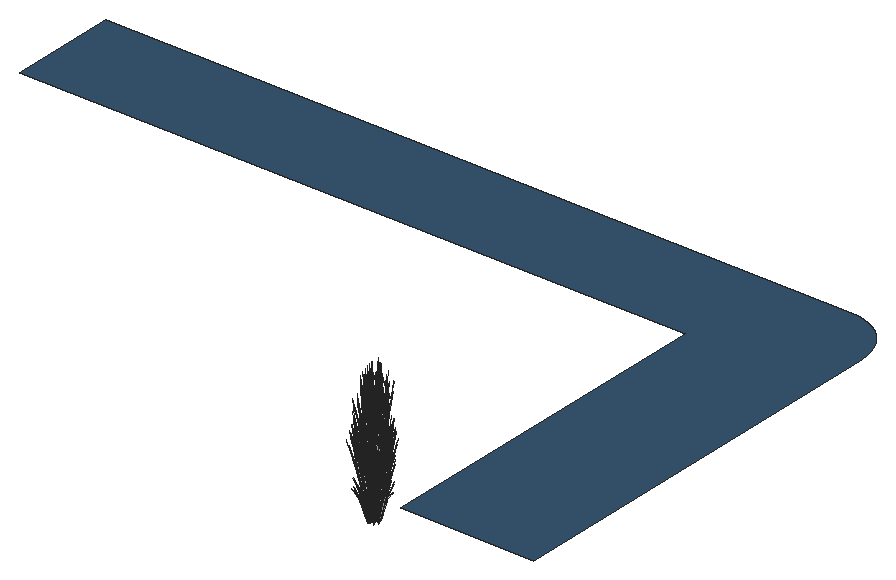
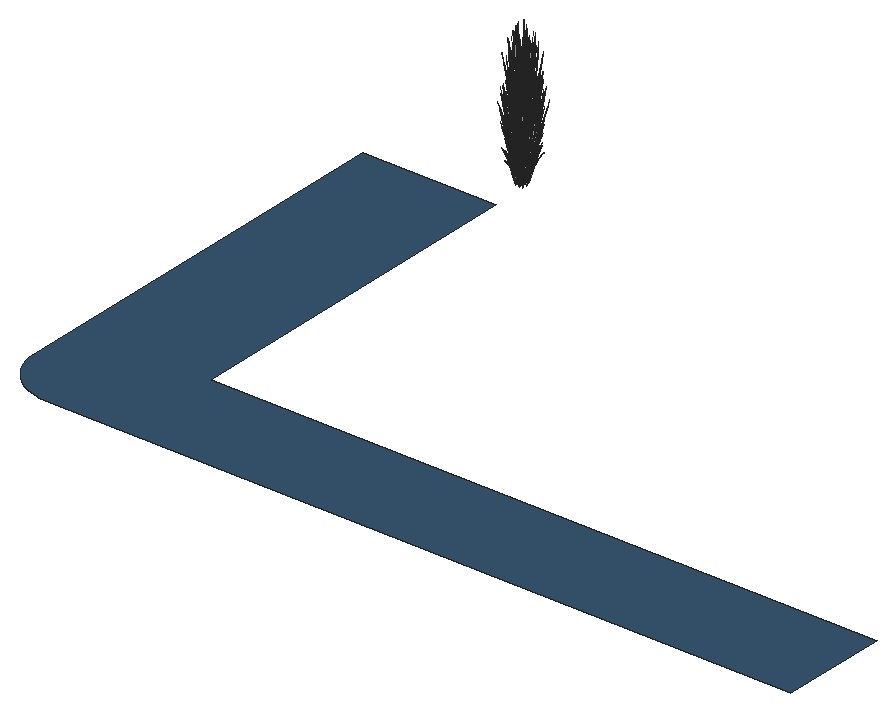
# SketchUp Ruby script. Lengths in inches.
U = 1.inch
M = Sketchup.active_model
def pt(a) = Geom::Point3d.new(a.map { |v| v * U })
def face(e, loops, mat)
  f = e.add_face(loops[0].map { |a| pt(a) })
  loops[1..].each { |l| e.add_face(l.map { |a| pt(a) }).erase! }
  f.material = f.back_material = mat if mat
  f
end
# faces: each face lists its corners as indices into pts; further lists are holes
def faces(e, pts, list, mat = nil) = list.each { |f| face(e, (f[0].is_a?(Array) ? f : [f]).map { |l| l.map { |i| pts[i] } }, mat) }
# xy, xz, yz: faces in a plane at the given z, y or x. An outline is a flat list of corners, or four numbers for a rectangle; further outlines are holes
def ring(l) = l.size == 4 ? [[l[0], l[1]], [l[2], l[1]], [l[2], l[3]], [l[0], l[3]]] : l.each_slice(2).to_a
def flat(e, list, mat, &to3) = list.each { |f| face(e, (f[0].is_a?(Array) ? f : [f]).map { |l| ring(l).map { |u, v| to3.(u, v) } }, mat) }
def xy(e, z, list, mat = nil) = flat(e, list, mat) { |x, y| [x, y, z] }
def xz(e, y, list, mat = nil) = flat(e, list, mat) { |x, z| [x, y, z] }
def yz(e, x, list, mat = nil) = flat(e, list, mat) { |y, z| [x, y, z] }
def lines(e, pts, list) = list.each { |a, b| e.add_line(pt(pts[a]), pt(pts[b])) }
# prism: a flat outline (further loops are holes) pulled along v
def prism(e, loops, v, mat = nil)
  f = face(e, loops, mat); d = Geom::Vector3d.new(v.map { |x| x * U })
  f.pushpull(f.normal.samedirection?(d) ? d.length : -d.length)
end
def box(e, o, s, mat = nil) = prism(e, [[o, [o[0] + s[0], o[1], o[2]], [o[0] + s[0], o[1] + s[1], o[2]], [o[0], o[1] + s[1], o[2]]]], [0, 0, s[2]], mat)
def at(x, y, z, deg = 0) = Geom::Transformation.translation(pt([x, y, z])) * Geom::Transformation.rotation(ORIGIN, Z_AXIS, deg.degrees)
def axes(o, x, y, z) = Geom::Transformation.new([*x, 0, *y, 0, *z, 0, *pt(o).to_a, 1])
def part(name) = M.definitions.add(name)
# library, detail: a bought-in or finely detailed component or shape, given as its bounding box
def library(name, o, s) = part(name).tap { |d| box(d.entities, o, s) }
def detail(e, o, s) = box(e.add_group.entities, o, s)
def put(e, d, t, mat = nil) = e.add_instance(d, t).tap { |i| i.material = mat if mat }
def group(e, t, mat = nil) = e.add_group.tap { |g| g.transformation = t; g.material = mat if mat }.entities
root = M.entities
M.materials.add("Carpet_04_1K").color = [56, 85, 112]
M.materials.add("LightPink_Translucent").color = [144, 107, 117]
M.materials["LightPink_Translucent"].alpha = 0.75
c1 = part("blade")
p = [[2.15,0.21,22],[0,0.17,0],[0.09,0.45,0],[2.18,0.31,22],[2.29,0.31,22],[0.38,0.45,0],
  [2.48,0.24,33],[2.49,0.24,33],[2.48,0.22,33]]
faces(c1.entities,p,[[0,1,2,3],[4,5,2,3],[6,3,4,7],[8,0,3,6]])
c2 = part("seeds")
p = [[0.3,-0.1,1.38],[-0.01,-0.03,1.59],[-0.01,-0.03,0.03],[0.14,-0.07,-0.07],[0.29,-0.03,3],[0.15,0.01,3.11]]
faces(c2.entities,p,[[0,1,2,3],[1,0,4,5]],"LightPink_Translucent")
c3 = part("blade with seeds")
put(c3.entities,c1,at(0,0,0))
put(c3.entities,c2,axes([2.4,0.25,30.99],[1.5799,-0.05474,1.17369],[-0.12525,1.92788,0.29478],[-0.07173,-0.02425,1.56792]))
xy(root,1398,[[330.57,637.9,390.57,637.9,390.57,822.7,390.37,825.83,389.76,828.91,388.75,831.89,387.36,834.7,385.62,837.3125,383.55,839.67,381.19,841.74,378.57,843.49,375.76,844.875,372.79,845.88,369.71,846.5,366.57,846.7,30.57,846.7,30.57,798.7,330.57,798.7]],"Carpet_04_1K")
put(root,c3,axes([332.43,620.08,1402.71],[-0.03584,0.03562,1.77383],[-0.35118,-0.12018,-0.16761],[-0.01271,-0.15545,0.31391]))
put(root,c3,axes([331.14,620.64,1402.68],[-0.34695,-0.11691,-0.51099],[0.11892,-0.40083,-0.3958],[-0.03181,-0.16138,0.97773]))
put(root,c3,axes([331.35,619.64,1400.77],[0.04528,0.27194,1.1486],[-0.25117,-0.15062,0.84392],[0.02703,-0.13924,0.25299]))
put(root,c3,axes([331.89,620.94,1402.68],[-0.25266,-0.31335,-0.51099],[0.2669,-0.27442,-0.3958],[0.03844,-0.15921,0.97773]))
put(root,c3,axes([330.52,619.4,1402.71],[-0.00658,0.0559,1.77383],[-0.32474,0.20287,-0.16761],[-0.09556,-0.1037,0.31391]))
put(root,c3,axes([330.45,620.39,1403.09],[0.39316,-0.11987,0.53763],[0.06823,0.47021,0.4433],[-0.09247,-0.13858,1.11249]))
put(root,c3,axes([331.34,620.48,1402.73],[0.34777,0.12192,0.48003],[-0.11892,0.40083,0.3958],[-0.0209,-0.15763,0.9933]))
put(root,c3,axes([331.4375,620.62,1403.03],[-0.34538,0.21713,-0.1216],[-0.16972,-0.38536,-0.67495],[-0.04557,-0.16239,1.02557]))
put(root,c3,axes([332.15,621.11,1403.03],[-0.3879,-0.02311,-0.1216],[0.0106,-0.43749,-0.67495],[0.02694,-0.1685,1.02557]))
put(root,c3,axes([332.13,620.83,1402.53],[0.23881,-0.24554,-0.35414],[0.22606,0.28036,0.4572],[0.0344,-0.14245,0.87481]))
put(root,c3,axes([330.0625,619.96,1400.77],[0.18411,0.16231,1.1486],[-0.26813,0.09757,0.84392],[-0.05737,-0.12474,0.25299]))
put(root,c3,axes([331.43,620.45,1402.73],[0.26007,-0.1585,0.0643],[0.12729,0.28902,0.50621],[-0.02512,-0.1274,0.77189]))
put(root,c3,axes([330.51,620.82,1402.98],[-0.30095,-0.22541,-0.71045],[0.21388,-0.395,0.08574],[-0.10904,-0.13459,1.00501]))
put(root,c3,axes([330.4,620.52,1402.53],[-0.05451,-0.37564,-0.35414],[0.31161,-0.09919,0.4572],[-0.0837,-0.10765,0.87481]))
put(root,c3,axes([330.54,620.49,1402.73],[0.16041,-0.29625,0.0643],[0.22843,0.17248,0.50621],[-0.07385,-0.09498,0.77189]))
put(root,c3,axes([329.92,620.45,1399.49],[-0.03419,0.06144,1.76342],[-0.3455,0.13246,-0.26939],[-0.08346,-0.12049,0.30037]))
put(root,c3,axes([330.49,622.14,1400.1],[-0.14494,-0.47823,-0.69835],[0.41752,-0.17223,-0.18329],[-0.01602,-0.16194,1.54149]))
put(root,c3,axes([329.73,621.07,1401.875],[0.1311,0.08035,1.71376],[-0.27131,0.33708,0.13857],[-0.16909,-0.15206,0.73262]))
put(root,c3,axes([332.43,620.68,1399.49],[-0.05283,-0.03674,1.76342],[-0.13569,-0.41045,-0.26939],[0.09154,-0.11138,0.30037]))
put(root,c3,axes([331.33,620.77,1403.05],[-0.1064,0.35863,0.35414],[-0.31043,-0.1046,-0.4572],[-0.02846,-0.14439,0.87481]))
put(root,c3,axes([330.37,620.83,1402.68],[-0.34827,0.11086,-0.51099],[-0.06092,-0.41983,-0.3958],[-0.09354,-0.12031,0.97773]))
put(root,c3,axes([332.125,620.92,1402.73],[0.25132,0.3182,0.48003],[-0.2669,0.27442,0.3958],[0.04636,-0.14929,0.9933]))
put(root,c3,axes([330.61,620.46,1403.43],[-0.23555,0.44708,-0.13619],[-0.34112,-0.25757,-0.75594],[-0.11858,-0.12631,1.14864]))
put(root,c3,axes([332.22,620.95,1402.73],[0.29004,0.02173,0.0643],[-0.00795,0.32812,0.50621],[0.03035,-0.12569,0.77189]))
put(root,c3,axes([332,621.17,1403.05],[-0.23881,0.24554,0.35414],[-0.22606,-0.28036,-0.4572],[0.0344,-0.14245,0.87481]))
put(root,c3,axes([332.42,621.84,1402.98],[0.18436,-0.36797,-0.71045],[0.32306,0.26151,0.08574],[0.11008,-0.13332,1.00501]))
put(root,c3,axes([330.43,620.76,1400.375],[-0.22066,-0.46731,0],[0.36918,-0.26061,-0.51607],[0.08408,-0.05936,1.63711]))
put(root,c3,axes([332.41,621.66,1402.68],[-0.09067,-0.42583,-0.51099],[0.34336,-0.07449,-0.3958],[0.0984,-0.11438,0.97773]))
put(root,c3,axes([330.92,620.2,1400.13],[-0.2439,0.26754,-0.03893],[-0.22348,-0.29302,-0.17649],[-0.01573,-0.08303,0.58215]))
put(root,c3,axes([329.71,620.33,1402.72],[-0.07594,-0.00329,1.74944],[-0.24177,0.32918,-0.27667],[-0.129,-0.06726,0.14031]))
put(root,c3,axes([332.58,621.97,1403.03],[-0.32648,-0.25715,-0.1216],[0.18809,-0.3724,-0.67495],[0.09224,-0.12945,1.02557]))
put(root,c3,axes([331.23,623.37,1401.33],[0.305,0.18805,1.51261],[-0.29879,0.40513,0.59816],[-0.13384,-0.24012,1.26806]))
put(root,c3,axes([330.59,620.83,1403.05],[0.05451,0.37564,0.35414],[-0.31161,0.09919,-0.4572],[-0.0837,-0.10765,0.87481]))
put(root,c3,axes([329.63,622.07,1400.02],[0,-0.46636,-0.49651],[0.39487,0,0],[0,-0.10622,1.57504]))
put(root,c3,axes([330.73,620.69,1400.02],[0.33032,-0.23318,-0.49651],[0.19744,0.41812,0],[0.07523,-0.05311,1.57504]))
put(root,c3,axes([332.69,621.5,1400.59],[-0.12609,-0.01381,1.43002],[-0.12917,-0.37055,-0.30754],[0.1549,-0.10482,0.61141]))
put(root,c3,axes([329.65,621.08,1403.09],[0.29147,-0.34417,0.53763],[0.25138,0.3655,0.4433],[-0.13675,-0.06349,1.11249]))
put(root,c3,axes([333.38,621.86,1402.71],[-0.0461,-0.00354,1.77383],[-0.19143,-0.37951,-0.16761],[0.07688,-0.12478,0.31391]))
put(root,c3,axes([331.12,621.65,1400.06],[0.23773,-0.35053,-0.62353],[0.29532,0.31785,-0.16365],[0.09526,-0.08744,1.37633]))
put(root,c3,axes([332.84,620.82,1400.77],[-0.11756,0.2374,1.1486],[-0.10105,-0.31895,0.84392],[0.09709,-0.07992,0.25299]))
put(root,c3,axes([332.67,621.71,1402.53],[0.30722,-0.06665,-0.35414],[0.08112,0.381,0.4572],[0.08804,-0.10234,0.87481]))
put(root,c3,axes([329.78,621.07,1402.73],[0.01777,-0.35463,0.0643],[0.26836,0.00972,0.50621],[-0.1028,-0.03711,0.77189]))
put(root,c3,axes([330.71,622.26,1400.21],[0.17124,-0.42022,-0.44739],[0.35581,0.20224,0.21531],[0,-0.09687,1.43643]))
put(root,c3,axes([329.68,621.19,1402.53],[-0.20082,-0.29199,-0.35414],[0.2293,-0.2764,0.4572],[-0.1165,-0.04206,0.87481]))
put(root,c3,axes([330.86,622.06,1400.67],[-0.04113,-0.53214,-0.29095],[0.42835,-0.03218,-0.50002],[0.07543,-0.07088,1.59708]))
put(root,c3,axes([329.8,622.08,1400.03],[0.24637,-0.29097,-0.30978],[0.24637,0.29097,0.30978],[0,-0.09372,1.38974]))
put(root,c3,axes([329.7,620.6875,1400.13],[-0.10181,0.3808,-0.03893],[-0.31336,-0.11714,-0.17649],[-0.04758,-0.06228,0.58215]))
put(root,c3,axes([332.42,621.93,1403.05],[-0.30722,0.06665,0.35414],[-0.08112,-0.381,-0.4572],[0.08804,-0.10234,0.87481]))
put(root,c3,axes([330.67,622.61,1400.67],[-0.39748,-0.22252,-0.29095],[0.19139,-0.46966,-0.50002],[-0.01249,-0.11531,1.59708]))
put(root,c3,axes([329.53,622.43,1400.375],[-0.44133,0,0],[0,-0.52122,-0.51607],[0,-0.11871,1.63711]))
put(root,c3,axes([329.61,621.5,1400.59],[0.06891,0.12984,1.43002],[-0.15879,0.35293,-0.30754],[-0.16304,-0.08436,0.61141]))
put(root,c3,axes([330.81,620.875,1400.03],[0.32928,0.11539,-0.30978],[-0.08291,0.40636,0.30978],[0.06638,-0.04686,1.38974]))
put(root,c3,axes([329.89,621.38,1402.98],[-0.35281,-0.01123,-0.71045],[0.0237,-0.47284,0.08574],[-0.14947,-0.0499,1.00501]))
put(root,c3,axes([332.7,621.875,1402.73],[0.2423,0.19613,0.0643],[-0.14107,0.2793,0.50621],[0.07768,-0.0903,0.77189]))
put(root,c3,axes([332.63,621.79,1402.73],[0.08753,0.42921,0.48003],[-0.34336,0.07449,0.3958],[0.1012,-0.10094,0.9933]))
put(root,c3,axes([333.55,622.3125,1402.72],[0.04898,-0.07104,1.74944],[-0.06269,-0.43574,-0.27667],[0.12289,-0.08262,0.14031]))
put(root,c3,axes([329.875,622.29,1400.33],[-0.32829,0.39208,0.30756],[-0.32849,-0.38796,-0.36492],[-0.01146,-0.11134,1.64885]))
put(root,c3,axes([329.42,620.61,1402.71],[0.02617,0.04654,1.77383],[-0.12614,0.41836,-0.16761],[-0.12775,0.00303,0.31391]))
put(root,c3,axes([330.92,622.47,1400.43],[0.39767,0.22603,0.24065],[-0.19139,0.46966,0.50002],[0,-0.10827,1.60543]))
put(root,c3,axes([330.77,623.11,1400.4375],[0.09355,-0.55261,-0.23429],[0.44354,0.09633,0.51271],[-0.0775,-0.07631,1.5644]))
put(root,c3,axes([329.78,621.48,1402.68],[-0.25628,0.30892,-0.51099],[-0.22444,-0.32634,-0.3958],[-0.13021,-0.047,0.97773]))
put(root,c3,axes([329.97,621.34,1403.05],[0.20082,0.29199,0.35414],[-0.2293,0.2764,-0.4572],[-0.1165,-0.04206,0.87481]))
put(root,c3,axes([329.2,621.89,1400.77],[0.22533,-0.03337,1.1486],[-0.14293,0.29403,0.84392],[-0.11135,-0.04411,0.25299]))
put(root,c3,axes([330.79,622.16,1400.72],[-0.38326,0.02879,0.44739],[-0.03466,-0.47788,-0.21531],[0.06861,-0.04843,1.43643]))
put(root,c3,axes([329.91,621.15,1403.03],[-0.0189,0.47427,-0.1216],[-0.35781,-0.01296,-0.67495],[-0.13781,-0.03295,1.02557]))
put(root,c3,axes([329.8,622.51,1400.48],[0,0.46636,0.49651],[-0.39487,0,0],[0,-0.10622,1.57504]))
put(root,c3,axes([332.59,622.97,1403.03],[-0.17758,-0.42229,-0.1216],[0.31518,-0.20752,-0.67495],[0.13282,-0.05572,1.02557]))
put(root,c3,axes([332.57,622.61,1402.68],[0.09562,-0.42421,-0.51099],[0.32782,0.1454,-0.3958],[0.13199,-0.0389,0.97773]))
put(root,c3,axes([332.06,620.88,1400.375],[0.22066,-0.46731,0],[0.36918,0.26061,-0.51607],[0.08408,0.05936,1.63711]))
put(root,c3,axes([329.46,621.81,1401.875],[0.14639,-0.01056,1.71376],[-0.09712,0.45778,0.13857],[-0.20862,-0.02831,0.73262]))
put(root,c3,axes([330.73,622.88,1400.21],[-0.21202,-0.39143,-0.44739],[0.32115,-0.27564,0.21531],[-0.06861,-0.04843,1.43643]))
put(root,c3,axes([330.78,622.33,1400.36],[0.15345,0.52148,0.45755],[-0.43845,0.18134,0.17955],[0.00536,-0.09582,1.58856]))
put(root,c3,axes([332.92,622.73,1399.98],[-0.22732,0.05597,1.41583],[-0.03618,-0.44548,0.08104],[0.15921,-0.06743,0.80566]))
put(root,c3,axes([333.34,622.33,1400.26],[-0.21881,-0.29821,-0.06488],[0.23965,-0.27324,-0.29416],[0.0679,-0.01924,0.97024]))
put(root,c3,axes([330.7,622.74,1400.72],[-0.17124,0.42022,0.44739],[-0.35581,-0.20224,-0.21531],[0,-0.09687,1.43643]))
put(root,c3,axes([331.33,622.375,1400.21],[0,-0.53961,0],[0.44133,0,0],[0,0,1.79456]))
put(root,c3,axes([331.87,621.125,1400.48],[-0.33032,-0.23318,0.49651],[0.19744,-0.41812,0],[0.07523,0.05311,1.57504]))
put(root,c3,axes([332.51,622.76,1402.98],[0.31014,-0.20596,-0.71045],[0.17284,0.42397,0.08574],[0.14985,-0.04816,1.00501]))
put(root,c3,axes([330.54,623.03,1400.06],[-0.36714,-0.07646,-0.62353],[0.07747,-0.47163,-0.16365],[-0.10956,-0.05715,1.37633]))
put(root,c3,axes([331.12,622.03,1400.36],[-0.29264,0.42323,0.45755],[-0.34767,-0.3736,0.17955],[0.07055,-0.04224,1.58856]))
put(root,c3,axes([331.44,622.79,1400.3],[-0.32829,-0.4014,-0.06131],[0.32849,-0.40164,0],[-0.01146,-0.01402,1.75571]))
put(root,c3,axes([330.61,621.34,1400.47],[-0.10196,0.46348,0.17642],[-0.3731,-0.13116,0.35086],[0.06445,-0.00226,1.60407]))
put(root,c3,axes([332.47,622.85,1403.05],[-0.29332,-0.1301,0.35414],[0.08555,-0.37955,-0.4572],[0.11809,-0.0348,0.87481]))
put(root,c3,axes([329.4,622.15,1402.73],[0.09971,-0.42522,0.48003],[0.32782,0.1454,0.3958],[-0.12892,0.02555,0.9933]))
put(root,c3,axes([330.46,621.71,1399.59],[-0.3474,0.18671,1.28929],[-0.11057,-0.53572,0.50096],[0.21332,0.00891,1.46642]))
put(root,c3,axes([331.39,621.85,1400.62],[0.06809,-0.4162,0.1448],[0.33266,0.07225,-0.41347],[0.06054,0.04274,1.26744]))
put(root,c3,axes([329.37,622.04,1402.73],[-0.12963,-0.31798,0.0643],[0.23638,-0.15564,0.50621],[-0.1042,0.03071,0.77189]))
put(root,c3,axes([330.82,622.84,1400.36],[0.44609,0.09826,0.45755],[-0.09078,0.55493,0.17955],[-0.06519,-0.05359,1.58856]))
put(root,c3,axes([333.17,622.4375,1399.49],[-0.01845,-0.0708,1.76342],[0.12793,-0.41416,-0.26939],[0.12905,-0.00596,0.30037]))
put(root,c3,axes([329.36,622.37,1399.49],[0.00895,0.0735,1.76342],[-0.18044,0.38382,-0.26939],[-0.12817,-0.01935,0.30037]))
put(root,c3,axes([331.25,621.96,1400.72],[-0.21202,-0.39143,0.44739],[0.32115,-0.27564,-0.21531],[0.06861,0.04843,1.43643]))
put(root,c3,axes([330.15,623.75,1400.03],[-0.08291,-0.40636,-0.30978],[0.32928,-0.11539,0.30978],[-0.06638,-0.04686,1.38974]))
put(root,c3,axes([330.58,623.73,1400.47],[0.37926,-0.12378,0.17642],[0.09365,0.46065,0.35086],[-0.03382,-0.06712,1.60407]))
put(root,c3,axes([331.36,621.99,1400.67],[0.35635,-0.30962,-0.29095],[0.23697,0.43749,-0.50002],[0.08792,0.04443,1.59708]))
put(root,c3,axes([332.78,622.8,1402.53],[0.29332,0.1301,-0.35414],[-0.08555,0.37955,0.4572],[0.11809,-0.0348,0.87481]))
put(root,c3,axes([330.0625,623.92,1400.02],[-0.33032,-0.23318,-0.49651],[0.19744,-0.41812,0],[-0.07523,-0.05311,1.57504]))
put(root,c3,axes([332.26,621.16,1400.02],[0.33032,0.23318,-0.49651],[-0.19744,0.41812,0],[0.07523,0.05311,1.57504]))
put(root,c3,axes([329.33,622.2,1402.53],[-0.29332,-0.1301,-0.35414],[0.08555,-0.37955,0.4572],[-0.11809,0.0348,0.87481]))
put(root,c3,axes([331.63,622.49,1400.21],[0.39487,0,0],[0,0.48281,0],[0,0,1.78407]))
put(root,c3,axes([330.96,623.1,1400.67],[-0.35635,0.30962,-0.29095],[-0.23697,-0.43749,-0.50002],[-0.08792,-0.04443,1.59708]))
put(root,c3,axes([331.74,621.36,1400.47],[-0.37926,0.12378,0.17642],[-0.09365,-0.46065,0.35086],[0.03382,0.06712,1.60407]))
put(root,c3,axes([331.98,622.33,1401.875],[-0.14639,0.01056,1.71376],[0.09712,-0.45778,0.13857],[0.20862,0.02831,0.73262]))
put(root,c3,axes([332.17,621.34,1400.03],[0.08291,0.40636,-0.30978],[-0.32928,0.11539,0.30978],[0.06638,0.04686,1.38974]))
put(root,c3,axes([332.73,622.96,1402.73],[0.12963,0.31798,0.0643],[-0.23638,0.15564,0.50621],[0.1042,-0.03071,0.77189]))
put(root,c3,axes([331.5,622.25,1400.38],[-0.44609,-0.09826,0.49198],[0.09078,-0.55493,0.19306],[0.06519,0.05359,1.70813]))
put(root,c3,axes([332.71,622.85,1402.73],[-0.09971,0.42522,0.48003],[-0.32782,-0.1454,0.3958],[0.12892,-0.02555,0.9933]))
put(root,c3,axes([331.15,623.62,1400.2],[-0.11516,-0.40207,0],[0.32884,-0.1408,0],[0,0,1.54371]))
put(root,c3,axes([330.93,623.24,1400.62],[-0.06809,0.4162,0.1448],[-0.33266,-0.07225,-0.41347],[-0.06054,-0.04274,1.26744]))
put(root,c3,axes([329.64,622.16,1403.05],[0.29332,0.1301,0.35414],[-0.08555,0.37955,-0.4572],[-0.11809,0.0348,0.87481]))
put(root,c3,axes([331.58,623.5625,1400.18],[0.37054,-0.15823,-0.19198],[0.1302,0.45581,0.00008],[0.0409,-0.01749,1.73897]))
put(root,c3,axes([331.71,623.75,1400.47],[0.10196,-0.46348,0.17642],[0.3731,0.13116,0.35086],[-0.06445,0.00226,1.60407]))
put(root,c3,axes([331.62,622.7,1400.21],[0.24637,0.30123,0],[-0.24637,0.30123,0],[0,0,1.69266]))
put(root,c3,axes([330.22,622.14,1401.34],[0.10032,-0.06746,1.77064],[0.0346,0.47103,0.13857],[-0.2173,0.0625,0.63284]))
put(root,c3,axes([332.29,622.57,1400.47],[-0.2773,-0.3397,0.17642],[0.27945,-0.32949,0.35086],[-0.03063,0.06937,1.60407]))
put(root,c3,axes([331.78,622.06,1400.06],[0.36714,0.07646,-0.62353],[-0.07747,0.47163,-0.16365],[0.10956,0.05715,1.37633]))
put(root,c3,axes([333.4,622.88,1400.77],[-0.21807,0.07699,1.1486],[0.10265,-0.31819,0.84392],[0.11568,0.02177,0.25299]))
put(root,c3,axes([331.07,623.8,1400.2],[-0.35581,-0.20937,0],[0.17124,-0.43505,0],[0,0,1.62707]))
put(root,c3,axes([331.36,623.24,1400.46],[-0.34464,-0.37536,-0.25192],[0.29,-0.42149,0.5513],[-0.0928,0.04391,1.68216]))
put(root,c3,axes([330.45,623.96,1400.48],[0.33032,0.23318,0.49651],[-0.19744,0.41812,0],[-0.07523,-0.05311,1.57504]))
put(root,c3,axes([331.62,622.35,1400.72],[0.17124,-0.42022,0.44739],[0.35581,0.20224,-0.21531],[0,0.09687,1.43643]))
put(root,c3,axes([333.3,624.23,1402.71],[-0.03191,-0.04083,1.77383],[0.06981,-0.43764,-0.16761],[0.12571,-0.02796,0.31391]))
put(root,c3,axes([329.14,622.45,1402.72],[-0.05763,0.06055,1.74944],[0.0049,0.44239,-0.27667],[-0.13211,0.05753,0.14031]))
put(root,c3,axes([331.55,622.59,1400.29],[0,0.53934,-0.05637],[-0.44133,0,0],[0,0.01695,1.79368]))
put(root,c3,axes([329.53,622.39,1402.68],[-0.09562,0.42421,-0.51099],[-0.32782,-0.1454,-0.3958],[-0.13199,0.0389,0.97773]))
put(root,c3,axes([329.51,622.03,1403.03],[0.17758,0.42229,-0.1216],[-0.31518,0.20752,-0.67495],[-0.13282,0.05572,1.02557]))
put(root,c3,axes([331.58,622.21,1400.21],[0.21202,0.39143,-0.44739],[-0.32115,0.27564,0.21531],[0.06861,0.04843,1.43643]))
put(root,c3,axes([333.02,623.86,1401.93],[-0.06755,-0.39203,-0.03492],[0.31928,-0.09013,-0.15832],[0.06667,0.02485,0.52218]))
put(root,c3,axes([330.26,624.21,1400.375],[-0.22066,0.46731,0],[-0.36918,-0.26061,-0.51607],[-0.08408,-0.05936,1.63711]))
put(root,c3,axes([332.19,623.85,1403.03],[0.0189,-0.47427,-0.1216],[0.35781,0.01296,-0.67495],[0.13781,0.03295,1.02557]))
put(root,c3,axes([332.52,622.58,1400.48],[0,-0.46636,0.49651],[0.39487,0,0],[0,0.10622,1.57504]))
put(root,c3,axes([331.53,622.93,1400.72],[0.38326,-0.02879,0.44739],[0.03466,0.47788,-0.21531],[-0.06861,0.04843,1.43643]))
put(root,c3,axes([331.77,622.44,1400.62],[0.32884,-0.136,0.1448],[0.11516,0.38837,-0.41347],[0,0.08547,1.26744]))
put(root,c3,axes([332.14,623.66,1403.05],[-0.20082,-0.29199,0.35414],[0.2293,-0.2764,-0.4572],[0.1165,0.04206,0.87481]))
put(root,c3,axes([331.1875,623.16,1400.21],[-0.38326,0.02879,-0.44739],[-0.03466,-0.47788,0.21531],[-0.06861,0.04843,1.43643]))
put(root,c3,axes([332.99,623.39,1400.59],[-0.085,-0.1147,1.43002],[0.1106,-0.37943,-0.30754],[0.17198,0.0514,0.61141]))
put(root,c3,axes([331.47,623.81,1400.2],[0.35581,0.20937,0],[-0.17124,0.43505,0],[0,0,1.74954]))
put(root,c3,axes([332.5,623.57,1402.72],[0.07571,-0.00789,1.74944],[0.20767,-0.36231,-0.27667],[0.13467,0.04783,0.14031]))
put(root,c3,axes([331.61,624.27,1400.19],[-0.21791,-0.46895,-0.05142],[0.36918,-0.26061,0.51607],[-0.09097,0.04465,1.6363]))
put(root,c3,axes([331.53,623.14,1400.62],[0.26075,0.2802,0.1448],[-0.2175,0.31612,-0.41347],[-0.06054,0.04274,1.26744]))
put(root,c3,axes([329.47,623.21,1402.73],[-0.08753,-0.42921,0.48003],[0.34336,-0.07449,0.3958],[-0.1012,0.10094,0.9933]))
put(root,c3,axes([329.41,623.13,1402.73],[-0.2423,-0.19613,0.0643],[0.14107,-0.2793,0.50621],[-0.07768,0.0903,0.77189]))
put(root,c3,axes([329.52,622.61,1401.875],[0.12246,-0.09864,1.71376],[0.1031,0.45582,0.13857],[-0.19225,0.10302,0.73262]))
put(root,c3,axes([332.21,623.62,1402.98],[0.35281,0.01123,-0.71045],[-0.0237,0.47284,0.08574],[0.14947,0.0499,1.00501]))
put(root,c3,axes([331.8125,624,1400.48],[0.33032,-0.23318,0.49651],[0.19744,0.41812,0],[-0.07523,0.05311,1.57504]))
put(root,c3,axes([331.34,623.63,1400.29],[0.15345,0.53576,-0.06012],[-0.43845,0.18773,0],[0.00536,0.01871,1.72173]))
put(root,c3,axes([331.51,624.21,1400.03],[-0.32928,-0.11539,-0.30978],[0.08291,-0.40636,0.30978],[-0.06638,0.04686,1.38974]))
put(root,c3,axes([329.14,623.39,1400.59],[0.12266,0.03828,1.43002],[0.07906,0.39104,-0.30754],[-0.16661,0.0732,0.61141]))
put(root,c3,axes([329.6875,623.07,1403.05],[0.30722,-0.06665,0.35414],[0.08112,0.381,-0.4572],[-0.08804,0.10234,0.87481]))
put(root,c3,axes([332.78,622.66,1400.375],[0.44133,0,0],[0,0.52122,-0.51607],[0,0.11871,1.63711]))
put(root,c3,axes([328.5,622.9,1402.71],[0.04504,0.01251,1.77383],[0.13934,0.41205,-0.16761],[-0.0922,0.10815,0.31391]))
put(root,c3,axes([332.61,622.93,1400.2],[-0.44111,-0.00373,-0.04976],[0,-0.52122,0.49943],[-0.01386,0.11865,1.58352]))
put(root,c3,axes([331.65,622.48,1400.67],[0.39748,0.22252,-0.29095],[-0.19139,0.46966,-0.50002],[0.01249,0.11531,1.59708]))
put(root,c3,axes([328.88,624.21,1400.77],[0.14709,-0.21136,1.1486],[0.05804,0.3346,0.84392],[-0.1063,0.05991,0.25299]))
put(root,c3,axes([332.42,623.82,1402.53],[0.20082,0.29199,-0.35414],[-0.2293,0.2764,0.4572],[0.1165,0.04206,0.87481]))
put(root,c3,axes([332.52,623.01,1400.03],[-0.24637,0.29097,-0.30978],[-0.24637,-0.29097,0.30978],[0,0.09372,1.38974]))
put(root,c3,axes([331.46,623.03,1400.67],[0.04113,0.53214,-0.29095],[-0.42835,0.03218,-0.50002],[-0.07543,0.07088,1.59708]))
put(root,c3,axes([332.32,623.93,1402.73],[-0.01777,0.35463,0.0643],[-0.26836,-0.00972,0.50621],[0.1028,0.03711,0.77189]))
put(root,c3,axes([331.61,622.83,1400.21],[-0.17124,0.42022,-0.44739],[-0.35581,-0.20224,0.21531],[0,0.09687,1.43643]))
put(root,c3,axes([329.43,623.29,1402.53],[-0.30722,0.06665,-0.35414],[-0.08112,-0.381,0.4572],[-0.08804,0.10234,0.87481]))
put(root,c3,axes([332.34,623.82,1402.73],[-0.26024,0.30729,0.48003],[-0.22444,-0.32634,0.3958],[0.1221,0.05668,0.9933]))
put(root,c3,axes([328.99,624.15,1403.65],[0.31145,0.12449,-0.06488],[-0.0958,0.38314,-0.29416],[-0.05094,0.05817,0.97024]))
put(root,c3,axes([331.2,623.44,1400.06],[-0.23773,0.35053,-0.62353],[-0.29532,-0.31785,-0.16365],[-0.09526,0.08744,1.37633]))
put(root,c3,axes([331.52,624.17,1403.05],[-0.05451,-0.37564,0.35414],[0.31161,-0.09919,-0.4572],[0.0837,0.10765,0.87481]))
put(root,c3,axes([331.62,624.03,1400.33],[0.44186,0.15158,0.30756],[-0.11054,0.54181,-0.36492],[-0.07313,0.06781,1.64885]))
put(root,c3,axes([331.59,624.4,1400.02],[-0.33032,0.23318,-0.49651],[-0.19744,-0.41812,0],[-0.07523,0.05311,1.57504]))
put(root,c3,axes([332.6875,623.02,1400.02],[0,0.46636,-0.49651],[-0.39487,0,0],[0,0.10622,1.57504]))
put(root,c3,axes([331.7,623.07,1401.875],[-0.1311,-0.08035,1.71376],[0.27131,-0.33708,0.13857],[0.16909,0.15206,0.73262]))
put(root,c3,axes([331.72,622.01,1402.47],[-0.30498,-0.24231,1.38283],[0.32203,-0.37727,0.59665],[0.0984,0.22736,1.33663]))
put(root,c3,axes([329.53,623.03,1403.03],[0.32648,0.25715,-0.1216],[-0.18809,0.3724,-0.67495],[-0.09224,0.12945,1.02557]))
put(root,c3,axes([332.18,623.98,1400.77],[-0.19872,-0.13409,1.1486],[0.2566,-0.13625,0.84392],[0.06921,0.11541,0.25299]))
put(root,c3,axes([331.49,624.37,1403.03],[0.21031,-0.39918,-0.1216],[0.30457,0.22997,-0.67495],[0.10587,0.11278,1.02557]))
put(root,c3,axes([329.97,622.92,1401.875],[0.08815,-0.14329,1.71376],[0.22258,0.38678,0.13857],[-0.15267,0.17614,0.73262]))
put(root,c3,axes([329.6875,623.34,1402.68],[0.09067,0.42583,-0.51099],[-0.34336,0.07449,-0.3958],[-0.0984,0.11438,0.97773]))
put(root,c3,axes([330.1,623.83,1403.05],[0.23881,-0.24554,0.35414],[0.22606,0.28036,-0.4572],[-0.0344,0.14245,0.87481]))
put(root,c3,axes([331.89,624.32,1400.375],[0.22066,0.46731,0],[-0.36918,0.26061,-0.51607],[-0.08408,0.05936,1.63711]))
put(root,c3,axes([331.21,624.7,1402.71],[0.00104,-0.05646,1.77383],[0.30246,-0.2491,-0.16761],[0.10506,0.08891,0.31391]))
put(root,c3,axes([332.24,624.48,1399.49],[0.02571,-0.06733,1.76342],[0.32373,-0.19829,-0.26939],[0.09815,0.10263,0.30037]))
put(root,c3,axes([331.7,622.47,1400.84],[-0.00964,-0.43909,1.41272],[0.43635,0.11382,0.59816],[-0.1032,0.24027,1.3335]))
put(root,c3,axes([331.8125,622.95,1400.09],[0.12941,0.42699,-0.69212],[-0.37279,0.15378,-0.18165],[0.0143,0.14459,1.52773]))
put(root,c3,axes([329.88,624.05,1402.73],[-0.29004,-0.02173,0.0643],[0.00795,-0.32812,0.50621],[-0.03035,0.12569,0.77189]))
put(root,c3,axes([329.27,624.42,1399.49],[0.04734,0.04659,1.76342],[0.08027,0.4317,-0.26939],[-0.10492,0.09206,0.30037]))
put(root,c3,axes([329.98,624.08,1402.73],[-0.25132,-0.3182,0.48003],[0.2669,-0.27442,0.3958],[-0.04636,0.14929,0.9933]))
put(root,c3,axes([331.74,624.17,1402.68],[0.34827,-0.11086,-0.51099],[0.06092,0.41983,-0.3958],[0.09354,0.12031,0.97773]))
put(root,c3,axes([330.77,624.23,1403.05],[0.1064,-0.35863,0.35414],[0.31043,0.1046,-0.4572],[0.02846,0.14439,0.87481]))
put(root,c3,axes([332.22,624.59,1400.67],[-0.22633,-0.01463,1.0506],[0.14947,-0.31064,0.58006],[0.08941,0.11036,0.8241]))
put(root,c3,axes([331.56,624.51,1402.73],[-0.16041,0.29625,0.0643],[-0.22843,-0.17248,0.50621],[0.07385,0.09498,0.77189]))
put(root,c3,axes([331.1875,625.51,1403.65],[0.2439,-0.26754,-0.06488],[0.22348,0.29302,-0.29416],[0.01573,0.08303,0.97024]))
put(root,c3,axes([331.63,624.43,1402.73],[-0.35104,0.10702,0.48003],[-0.06092,-0.41983,0.3958],[0.08256,0.12373,0.9933]))
put(root,c3,axes([329.9,623.27,1401.875],[0.06572,-0.16029,1.71376],[0.27569,0.33172,0.13857],[-0.12437,0.20675,0.73262]))
put(root,c3,axes([331.48,623.84,1400.59],[0.00623,-0.15459,1.43002],[0.29764,-0.17268,-0.30754],[0.09188,0.18503,0.61141]))
put(root,c3,axes([330.67,624.56,1402.73],[-0.26007,0.1585,0.0643],[-0.12729,-0.28902,0.50621],[0.02512,0.1274,0.77189]))
put(root,c3,axes([329.98,624.18,1402.53],[-0.23881,0.24554,-0.35414],[-0.22606,-0.28036,0.4572],[-0.0344,0.14245,0.87481]))
put(root,c3,axes([329.15,624.1,1402.72],[-0.00877,0.09229,1.74944],[0.24897,0.32105,-0.27667],[-0.06518,0.15182,0.14031]))
put(root,c3,axes([329.95,623.89,1403.4],[0.3879,0.02311,-0.13498],[-0.0106,0.43749,-0.74919],[-0.02694,0.1685,1.13838]))
put(root,c3,axes([330.67,624.38,1403.03],[0.34538,-0.21713,-0.1216],[0.16972,0.38536,-0.67495],[0.04557,0.16239,1.02557]))
put(root,c3,axes([330.77,624.53,1403.0625],[-0.34777,-0.12192,0.53283],[0.11892,-0.40083,0.43934],[0.0209,0.15763,1.10256]))
put(root,c3,axes([330.13,625.13,1400.77],[-0.00913,-0.2773,1.1486],[0.22824,0.19778,0.84392],[-0.04489,0.13217,0.25299]))
put(root,c3,axes([330.73,624.47,1399.49],[0.05712,-0.02538,1.76342],[0.34359,0.13968,-0.26939],[0.01005,0.15742,0.30037]))
put(root,c3,axes([330.21,624.06,1403],[0.25266,0.31335,-0.5672],[-0.2669,0.27442,-0.43934],[-0.03844,0.15921,1.08528]))
put(root,c3,axes([329.9375,624.53,1400.82],[0.32063,-0.08258,0.06507],[0.07371,0.33271,-0.86304],[-0.02033,0.16842,0.7736]))
put(root,c3,axes([330.96,624.36,1402.68],[0.34695,0.11691,-0.51099],[-0.11892,0.40083,-0.3958],[0.03181,0.16138,0.97773]))
put(root,c3,axes([331.16,623.54,1401.875],[-0.08068,-0.14973,1.71376],[0.3728,-0.12606,0.13857],[0.08426,0.23506,0.73262]))
put(root,c3,axes([330.8,624.61,1402.53],[-0.1064,0.35863,-0.35414],[-0.31043,-0.1046,0.4572],[0.02846,0.14439,0.87481]))
put(root,c3,axes([330.13,623.92,1403.34],[-0.00918,0.43138,-0.7886],[-0.38672,-0.02897,0.09517],[-0.04081,0.18275,1.11556]))
put(root,c3,axes([329.125,625.05,1402.71],[0.04004,-0.02816,1.77383],[0.33095,0.18728,-0.16761],[-0.00778,0.15594,0.31391]))
put(root,c3,axes([330.5,623.61,1401.875],[-0.00864,-0.17899,1.71376],[0.37441,0.11874,0.13857],[-0.02316,0.25508,0.73262]))
put(root,c3,axes([330.84,624.29,1402.98],[0.16845,0.3792,-0.71045],[-0.34676,0.21133,0.08574],[0.03939,0.18322,1.00501]))
put(root,c3,axes([329.86,624.88,1400.59],[0.11138,-0.07357,1.43002],[0.27499,0.22183,-0.30754],[-0.08185,0.19194,0.61141]))
put(root,c3,axes([330.58,625.24,1402.72],[0.04474,0.0751,1.74944],[0.36104,0.0295,-0.27667],[0.03631,0.16562,0.14031]))
put(root,c3,axes([330.01,624.52,1401.36],[0.00775,-0.24075,1.54345],[0.34877,0.12716,0.21329],[-0.03022,0.25658,0.72882]))
